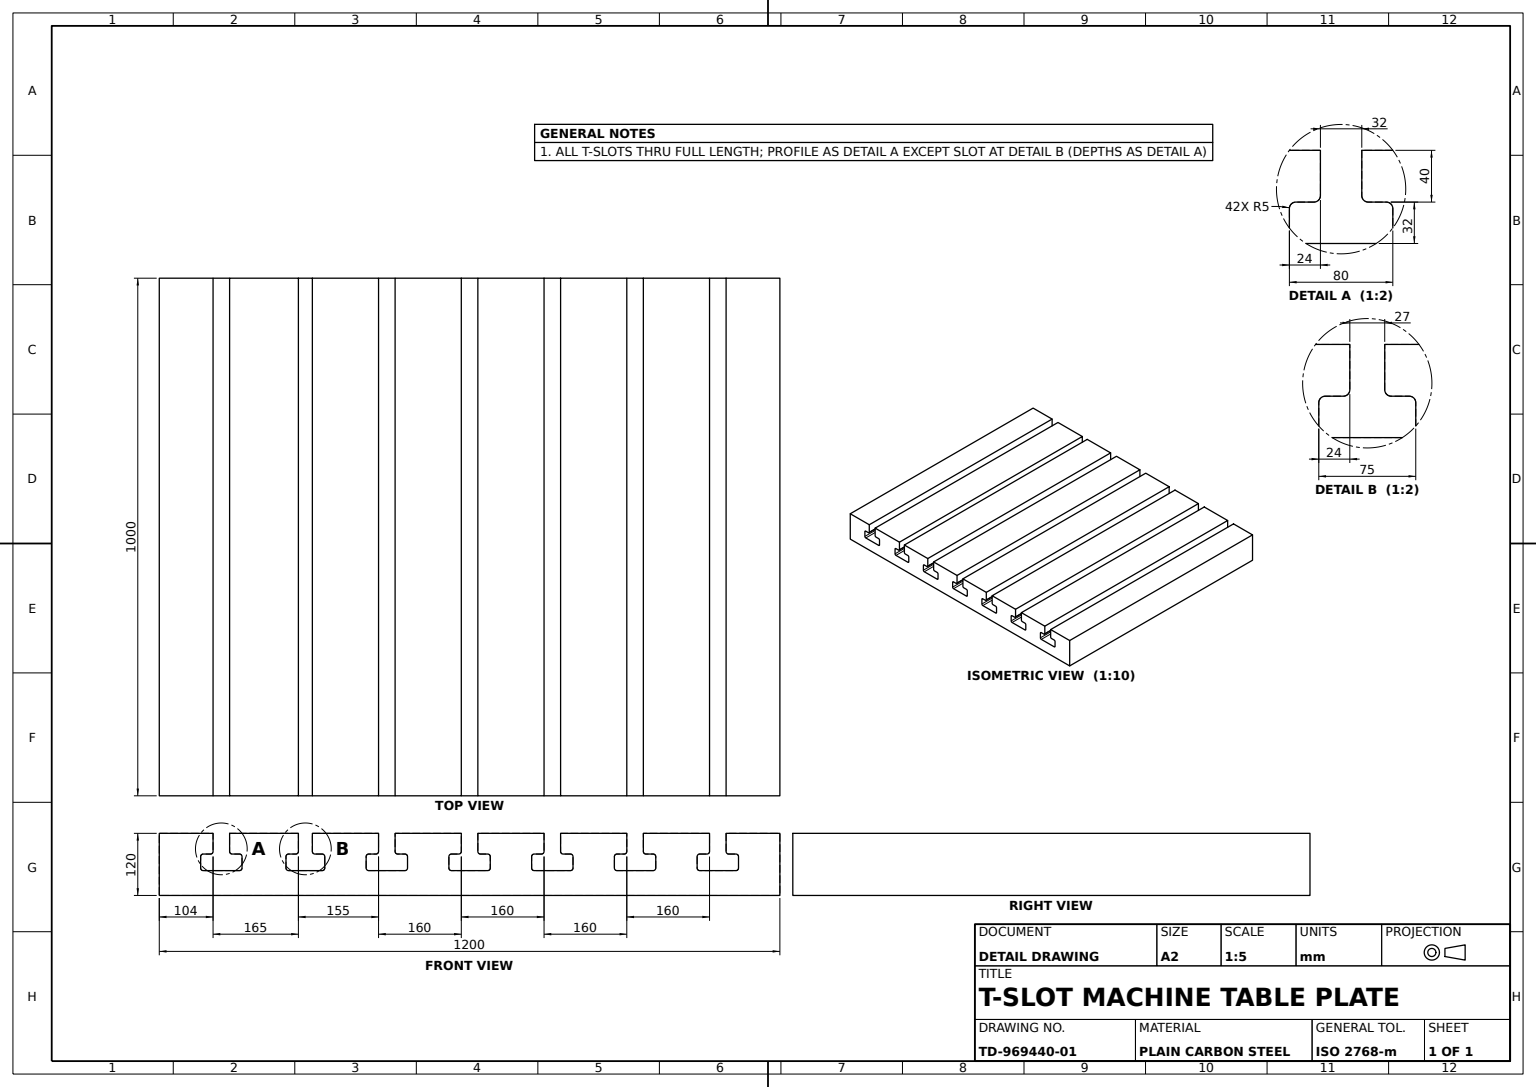
solid
v1 (104,1000,120)
v2 (104,1000,85)
e1 v1 v2 LINE
v3 (104,0,120)
e2 v1 v3 LINE
v4 (104,0,85)
e3 v3 v4 LINE
e4 v2 v4 LINE
face PLANE(AX(P(104,1000,0),D(-1,0,0),D(0,0,1))) rev [-e1 e2 e3 -e4]
v5 (1059,1000,80)
v6 (1059,0,80)
e5 v5 v6 LINE
v7 (1064,1000,85)
e6 v7 v5 CIRCLE(AX(P(1059,1000,85),D(0,1,0),D(0,0,-1)),5)
v8 (1064,0,85)
e7 v7 v8 LINE
e8 v8 v6 CIRCLE(AX(P(1059,0,85),D(0,1,0),D(0,0,-1)),5)
face CYL(AX(P(1059,1000,85),D(0,-1,0),D(0,0,-1)),5) [-e5 -e6 e7 e8]
v9 (885,1000,48)
v10 (885,0,48)
e9 v9 v10 LINE
v11 (955,0,48)
e10 v10 v11 LINE
v12 (955,1000,48)
e11 v12 v11 LINE
e12 v9 v12 LINE
face PLANE(AX(P(920,1000,48),D(0,0,-1),D(-1,0,0))) rev [e9 e10 -e11 -e12]
v13 (456,1000,85)
v14 (456,0,85)
e13 v13 v14 LINE
v15 (456,0,120)
e14 v14 v15 LINE
v16 (456,1000,120)
e15 v16 v15 LINE
e16 v13 v16 LINE
face PLANE(AX(P(456,1000,120),D(1,0,0),D(0,0,-1))) rev [e13 e14 -e15 -e16]
v17 (904,0,85)
v18 (899,0,80)
e17 v17 v18 CIRCLE(AX(P(899,0,85),D(0,1,0),D(0,0,-1)),5)
v19 (899,1000,80)
e18 v19 v18 LINE
v20 (904,1000,85)
e19 v20 v19 CIRCLE(AX(P(899,1000,85),D(0,1,0),D(0,0,-1)),5)
e20 v20 v17 LINE
face CYL(AX(P(899,1000,85),D(0,-1,0),D(0,0,-1)),5) [e17 -e18 -e19 e20]
v21 (85,0,80)
v22 (99,0,80)
e21 v21 v22 LINE
v23 (85,1000,80)
e22 v23 v21 LINE
v24 (99,1000,80)
e23 v23 v24 LINE
e24 v24 v22 LINE
face PLANE(AX(P(0,1000,80),D(0,0,-1),D(-1,0,0))) [-e21 -e22 e23 e24]
v25 (136,1000,85)
v26 (136,0,85)
e25 v25 v26 LINE
v27 (136,0,120)
e26 v27 v26 LINE
v28 (136,1000,120)
e27 v28 v27 LINE
e28 v28 v25 LINE
face PLANE(AX(P(136,1000,0),D(-1,0,0),D(0,0,1))) [e25 -e26 -e27 e28]
v29 (781,0,80)
v30 (776,0,85)
e29 v29 v30 CIRCLE(AX(P(781,0,85),D(0,1,0),D(0,0,1)),5)
v31 (776,1000,85)
e30 v31 v30 LINE
v32 (781,1000,80)
e31 v32 v31 CIRCLE(AX(P(781,1000,85),D(0,1,0),D(0,0,1)),5)
e32 v32 v29 LINE
face CYL(AX(P(781,1000,85),D(0,-1,0),D(0,0,-1)),5) [e29 -e30 -e31 e32]
v33 (904,1000,120)
e33 v33 v20 LINE
v34 (904,0,120)
e34 v33 v34 LINE
e35 v34 v17 LINE
face PLANE(AX(P(904,1000,85),D(-1,0,0),D(0,0,1))) rev [-e20 -e33 e34 e35]
v35 (936,1000,85)
v36 (936,1000,120)
e36 v35 v36 LINE
v37 (936,0,85)
e37 v35 v37 LINE
v38 (936,0,120)
e38 v37 v38 LINE
e39 v36 v38 LINE
face PLANE(AX(P(936,1000,120),D(1,0,0),D(0,0,-1))) rev [-e36 e37 e38 -e39]
v39 (1045,1000,48)
v40 (1045,0,48)
e40 v39 v40 LINE
v41 (1040,1000,53)
e41 v41 v39 CIRCLE(AX(P(1045,1000,53),D(0,-1,0),D(0,0,1)),5)
v42 (1040,0,53)
e42 v41 v42 LINE
e43 v42 v40 CIRCLE(AX(P(1045,0,53),D(0,-1,0),D(0,0,1)),5)
face CYL(AX(P(1045,1000,53),D(0,-1,0),D(0,0,-1)),5) rev [-e40 -e41 e42 e43]
v43 (424,1000,120)
v44 (424,0,120)
e44 v43 v44 LINE
v45 (424,0,85)
e45 v44 v45 LINE
v46 (424,1000,85)
e46 v46 v45 LINE
e47 v43 v46 LINE
face PLANE(AX(P(424,1000,120),D(-1,0,0),D(0,0,1))) rev [e44 e45 -e46 -e47]
v47 (776,0,120)
e48 v30 v47 LINE
v48 (776,1000,120)
e49 v48 v47 LINE
e50 v31 v48 LINE
face PLANE(AX(P(776,1000,120),D(1,0,0),D(0,0,-1))) rev [e30 e48 -e49 -e50]
e51 v24 v2 CIRCLE(AX(P(99,1000,85),D(0,-1,0),D(0,0,-1)),5)
e52 v22 v4 CIRCLE(AX(P(99,0,85),D(0,-1,0),D(0,0,-1)),5)
face CYL(AX(P(99,1000,85),D(0,-1,0),D(0,0,-1)),5) [-e24 e51 e4 -e52]
v49 (141,0,80)
v50 (155,0,80)
e53 v49 v50 LINE
v51 (141,1000,80)
e54 v51 v49 LINE
v52 (155,1000,80)
e55 v51 v52 LINE
e56 v52 v50 LINE
face PLANE(AX(P(0,1000,80),D(0,0,-1),D(-1,0,0))) [-e53 -e54 e55 e56]
v53 (0,0,0)
v54 (1200,0,0)
e57 v53 v54 LINE
v55 (0,1000,0)
e58 v55 v53 LINE
v56 (1200,1000,0)
e59 v56 v55 LINE
e60 v54 v56 LINE
face PLANE(AX(P(0,0,0),D(0,0,1),D(1,0,0))) rev [-e57 -e58 -e59 -e60]
v57 (160,1000,75)
v58 (160,0,75)
e61 v57 v58 LINE
v59 (160,1000,53)
e62 v59 v57 LINE
v60 (160,0,53)
e63 v59 v60 LINE
e64 v60 v58 LINE
face PLANE(AX(P(160,1000,0),D(1,0,0),D(0,0,-1))) rev [-e61 -e62 e63 e64]
v61 (960,1000,53)
e65 v12 v61 CIRCLE(AX(P(955,1000,53),D(0,-1,0),D(0,0,-1)),5)
v62 (960,0,53)
e66 v11 v62 CIRCLE(AX(P(955,0,53),D(0,-1,0),D(0,0,-1)),5)
e67 v61 v62 LINE
face CYL(AX(P(955,1000,53),D(0,-1,0),D(0,0,-1)),5) rev [-e65 e11 e66 -e67]
v63 (635,1000,48)
v64 (635,0,48)
e68 v63 v64 LINE
v65 (565,1000,48)
e69 v65 v63 LINE
v66 (565,0,48)
e70 v65 v66 LINE
e71 v66 v64 LINE
face PLANE(AX(P(600,1000,48),D(0,0,-1),D(-1,0,0))) rev [-e68 -e69 e70 e71]
v67 (955,0,80)
v68 (941,0,80)
e72 v67 v68 LINE
v69 (941,1000,80)
e73 v69 v68 LINE
v70 (955,1000,80)
e74 v70 v69 LINE
e75 v70 v67 LINE
face PLANE(AX(P(955,1000,80),D(0,0,1),D(1,0,0))) rev [e72 -e73 -e74 e75]
v71 (960,1000,75)
v72 (960,0,75)
e76 v71 v72 LINE
e77 v72 v67 CIRCLE(AX(P(955,0,75),D(0,-1,0),D(0,0,-1)),5)
e78 v71 v70 CIRCLE(AX(P(955,1000,75),D(0,-1,0),D(0,0,-1)),5)
face CYL(AX(P(955,1000,75),D(0,-1,0),D(0,0,-1)),5) rev [e76 e77 -e75 -e78]
v73 (640,0,53)
v74 (640,0,75)
e79 v73 v74 LINE
v75 (640,1000,75)
e80 v75 v74 LINE
v76 (640,1000,53)
e81 v76 v75 LINE
e82 v76 v73 LINE
face PLANE(AX(P(640,1000,53),D(1,0,0),D(0,0,-1))) rev [e79 -e80 -e81 e82]
e83 v57 v52 CIRCLE(AX(P(155,1000,75),D(0,-1,0),D(0,0,-1)),5)
e84 v58 v50 CIRCLE(AX(P(155,0,75),D(0,-1,0),D(0,0,-1)),5)
face CYL(AX(P(155,1000,75),D(0,-1,0),D(0,0,-1)),5) rev [-e56 -e83 e61 e84]
v77 (480,1000,53)
v78 (480,0,53)
e85 v77 v78 LINE
v79 (480,0,75)
e86 v78 v79 LINE
v80 (480,1000,75)
e87 v80 v79 LINE
e88 v77 v80 LINE
face PLANE(AX(P(480,1000,53),D(1,0,0),D(0,0,-1))) rev [e85 e86 -e87 -e88]
e89 v49 v26 CIRCLE(AX(P(141,0,85),D(0,1,0),D(0,0,-1)),5)
e90 v51 v25 CIRCLE(AX(P(141,1000,85),D(0,1,0),D(0,0,-1)),5)
face CYL(AX(P(141,1000,85),D(0,-1,0),D(0,0,-1)),5) [e54 e89 -e25 -e90]
v81 (795,1000,80)
v82 (795,0,80)
e91 v81 v82 LINE
e92 v82 v29 LINE
e93 v81 v32 LINE
face PLANE(AX(P(795,1000,80),D(0,0,1),D(1,0,0))) rev [e91 e92 -e32 -e93]
v83 (245,1000,75)
v84 (245,1000,53)
e94 v83 v84 LINE
v85 (245,0,75)
e95 v83 v85 LINE
v86 (245,0,53)
e96 v85 v86 LINE
e97 v84 v86 LINE
face PLANE(AX(P(245,1000,53),D(-1,0,0),D(0,0,1))) rev [-e94 e95 e96 -e97]
v87 (1045,0,80)
v88 (1040,0,75)
e98 v87 v88 CIRCLE(AX(P(1045,0,75),D(0,-1,0),D(0,0,-1)),5)
v89 (1040,1000,75)
e99 v89 v88 LINE
v90 (1045,1000,80)
e100 v90 v89 CIRCLE(AX(P(1045,1000,75),D(0,-1,0),D(0,0,-1)),5)
e101 v90 v87 LINE
face CYL(AX(P(1045,1000,75),D(0,-1,0),D(0,0,-1)),5) rev [e98 -e99 -e100 e101]
v91 (880,1000,75)
v92 (880,1000,53)
e102 v91 v92 LINE
v93 (880,0,75)
e103 v91 v93 LINE
v94 (880,0,53)
e104 v93 v94 LINE
e105 v92 v94 LINE
face PLANE(AX(P(880,1000,53),D(-1,0,0),D(0,0,1))) rev [-e102 e103 e104 -e105]
v95 (296,1000,120)
e106 v43 v95 LINE
v96 (296,0,120)
e107 v95 v96 LINE
e108 v96 v44 LINE
face PLANE(AX(P(0,0,120),D(0,0,1),D(1,0,0))) [-e44 e106 e107 e108]
v97 (885,0,80)
e109 v97 v93 CIRCLE(AX(P(885,0,75),D(0,-1,0),D(0,0,-1)),5)
v98 (885,1000,80)
e110 v98 v91 CIRCLE(AX(P(885,1000,75),D(0,-1,0),D(0,0,-1)),5)
e111 v98 v97 LINE
face CYL(AX(P(885,1000,75),D(0,-1,0),D(0,0,-1)),5) rev [e109 -e103 -e110 e111]
v99 (1115,1000,48)
v100 (1120,1000,53)
e112 v99 v100 CIRCLE(AX(P(1115,1000,53),D(0,-1,0),D(0,0,-1)),5)
v101 (1115,0,48)
e113 v99 v101 LINE
v102 (1120,0,53)
e114 v101 v102 CIRCLE(AX(P(1115,0,53),D(0,-1,0),D(0,0,-1)),5)
e115 v100 v102 LINE
face CYL(AX(P(1115,1000,53),D(0,-1,0),D(0,0,-1)),5) rev [-e112 e113 e114 -e115]
v103 (461,0,80)
e116 v103 v14 CIRCLE(AX(P(461,0,85),D(0,1,0),D(0,0,1)),5)
v104 (461,1000,80)
e117 v104 v13 CIRCLE(AX(P(461,1000,85),D(0,1,0),D(0,0,1)),5)
e118 v104 v103 LINE
face CYL(AX(P(461,1000,85),D(0,-1,0),D(0,0,-1)),5) [e116 -e13 -e117 e118]
v105 (0,0,120)
e119 v105 v53 LINE
v106 (0,1000,120)
e120 v106 v105 LINE
e121 v106 v55 LINE
face PLANE(AX(P(0,1000,120),D(1,0,0),D(0,0,-1))) rev [e58 -e119 -e120 e121]
v107 (80,1000,75)
v108 (80,0,75)
e122 v107 v108 LINE
e123 v23 v107 CIRCLE(AX(P(85,1000,75),D(0,-1,0),D(0,0,-1)),5)
e124 v21 v108 CIRCLE(AX(P(85,0,75),D(0,-1,0),D(0,0,-1)),5)
face CYL(AX(P(85,1000,75),D(0,-1,0),D(0,0,-1)),5) rev [-e122 -e123 e22 e124]
e125 v64 v73 CIRCLE(AX(P(635,0,53),D(0,-1,0),D(0,0,-1)),5)
e126 v63 v76 CIRCLE(AX(P(635,1000,53),D(0,-1,0),D(0,0,-1)),5)
face CYL(AX(P(635,1000,53),D(0,-1,0),D(0,0,-1)),5) rev [e68 e125 -e82 -e126]
v109 (584,0,120)
e127 v15 v109 LINE
v110 (584,1000,120)
e128 v110 v109 LINE
e129 v110 v16 LINE
face PLANE(AX(P(0,0,120),D(0,0,1),D(1,0,0))) [e15 e127 -e128 e129]
e130 v94 v10 CIRCLE(AX(P(885,0,53),D(0,-1,0),D(0,0,1)),5)
e131 v92 v9 CIRCLE(AX(P(885,1000,53),D(0,-1,0),D(0,0,1)),5)
face CYL(AX(P(885,1000,53),D(0,-1,0),D(0,0,-1)),5) rev [e105 e130 -e9 -e131]
v111 (800,1000,53)
v112 (800,1000,75)
e132 v111 v112 LINE
v113 (800,0,53)
e133 v111 v113 LINE
v114 (800,0,75)
e134 v113 v114 LINE
e135 v112 v114 LINE
face PLANE(AX(P(800,1000,53),D(1,0,0),D(0,0,-1))) rev [-e132 e133 e134 -e135]
v115 (1120,0,75)
v116 (1115,0,80)
e136 v115 v116 CIRCLE(AX(P(1115,0,75),D(0,-1,0),D(0,0,-1)),5)
v117 (1115,1000,80)
e137 v117 v116 LINE
v118 (1120,1000,75)
e138 v118 v117 CIRCLE(AX(P(1115,1000,75),D(0,-1,0),D(0,0,-1)),5)
e139 v118 v115 LINE
face CYL(AX(P(1115,1000,75),D(0,-1,0),D(0,0,-1)),5) rev [e136 -e137 -e138 e139]
v119 (725,1000,48)
v120 (725,0,48)
e140 v119 v120 LINE
v121 (795,0,48)
e141 v120 v121 LINE
v122 (795,1000,48)
e142 v122 v121 LINE
e143 v119 v122 LINE
face PLANE(AX(P(760,1000,48),D(0,0,-1),D(-1,0,0))) rev [e140 e141 -e142 -e143]
v123 (739,1000,80)
v124 (739,0,80)
e144 v123 v124 LINE
v125 (725,0,80)
e145 v124 v125 LINE
v126 (725,1000,80)
e146 v126 v125 LINE
e147 v123 v126 LINE
face PLANE(AX(P(725,1000,80),D(0,0,1),D(1,0,0))) rev [e144 e145 -e146 -e147]
v127 (1200,0,120)
v128 (1200,1000,120)
e148 v127 v128 LINE
e149 v127 v54 LINE
e150 v128 v56 LINE
face PLANE(AX(P(1200,0,120),D(-1,0,0),D(0,0,1))) rev [-e148 e149 e60 -e150]
v129 (405,1000,80)
v130 (405,0,80)
e151 v129 v130 LINE
v131 (400,0,75)
e152 v130 v131 CIRCLE(AX(P(405,0,75),D(0,-1,0),D(0,0,-1)),5)
v132 (400,1000,75)
e153 v132 v131 LINE
e154 v129 v132 CIRCLE(AX(P(405,1000,75),D(0,-1,0),D(0,0,-1)),5)
face CYL(AX(P(405,1000,75),D(0,-1,0),D(0,0,-1)),5) rev [e151 e152 -e153 -e154]
v133 (744,1000,120)
v134 (744,1000,85)
e155 v133 v134 LINE
v135 (744,0,120)
e156 v133 v135 LINE
v136 (744,0,85)
e157 v135 v136 LINE
e158 v134 v136 LINE
face PLANE(AX(P(744,1000,120),D(-1,0,0),D(0,0,1))) rev [-e155 e156 e157 -e158]
v137 (400,0,53)
e159 v131 v137 LINE
v138 (400,1000,53)
e160 v138 v137 LINE
e161 v132 v138 LINE
face PLANE(AX(P(400,1000,53),D(-1,0,0),D(0,0,1))) rev [e153 e159 -e160 -e161]
v139 (419,0,80)
e162 v45 v139 CIRCLE(AX(P(419,0,85),D(0,1,0),D(0,0,-1)),5)
v140 (419,1000,80)
e163 v140 v139 LINE
e164 v46 v140 CIRCLE(AX(P(419,1000,85),D(0,1,0),D(0,0,-1)),5)
face CYL(AX(P(419,1000,85),D(0,-1,0),D(0,0,-1)),5) [e162 -e163 -e164 e46]
v141 (475,1000,48)
e165 v141 v77 CIRCLE(AX(P(475,1000,53),D(0,-1,0),D(0,0,-1)),5)
v142 (475,0,48)
e166 v141 v142 LINE
e167 v142 v78 CIRCLE(AX(P(475,0,53),D(0,-1,0),D(0,0,-1)),5)
face CYL(AX(P(475,1000,53),D(0,-1,0),D(0,0,-1)),5) rev [-e165 e166 e167 -e85]
v143 (475,0,80)
e168 v143 v103 LINE
v144 (475,1000,80)
e169 v144 v104 LINE
e170 v144 v143 LINE
face PLANE(AX(P(475,1000,80),D(0,0,1),D(1,0,0))) rev [e168 -e118 -e169 e170]
v145 (720,1000,75)
v146 (720,0,75)
e171 v145 v146 LINE
v147 (720,0,53)
e172 v146 v147 LINE
v148 (720,1000,53)
e173 v148 v147 LINE
e174 v145 v148 LINE
face PLANE(AX(P(720,1000,53),D(-1,0,0),D(0,0,1))) rev [e171 e172 -e173 -e174]
e175 v140 v129 LINE
e176 v139 v130 LINE
face PLANE(AX(P(405,1000,80),D(0,0,1),D(1,0,0))) rev [-e151 -e175 e163 e176]
v149 (301,1000,80)
v150 (301,0,80)
e177 v149 v150 LINE
v151 (296,0,85)
e178 v150 v151 CIRCLE(AX(P(301,0,85),D(0,1,0),D(0,0,1)),5)
v152 (296,1000,85)
e179 v152 v151 LINE
e180 v149 v152 CIRCLE(AX(P(301,1000,85),D(0,1,0),D(0,0,1)),5)
face CYL(AX(P(301,1000,85),D(0,-1,0),D(0,0,-1)),5) [e177 e178 -e179 -e180]
e181 v40 v101 LINE
e182 v39 v99 LINE
face PLANE(AX(P(1080,1000,48),D(0,0,-1),D(-1,0,0))) rev [e40 e181 -e113 -e182]
e183 v112 v81 CIRCLE(AX(P(795,1000,75),D(0,-1,0),D(0,0,-1)),5)
e184 v114 v82 CIRCLE(AX(P(795,0,75),D(0,-1,0),D(0,0,-1)),5)
face CYL(AX(P(795,1000,75),D(0,-1,0),D(0,0,-1)),5) rev [-e183 e135 e184 -e91]
e185 v18 v97 LINE
e186 v19 v98 LINE
face PLANE(AX(P(885,1000,80),D(0,0,1),D(1,0,0))) rev [e18 e185 -e111 -e186]
e187 v125 v146 CIRCLE(AX(P(725,0,75),D(0,-1,0),D(0,0,1)),5)
e188 v126 v145 CIRCLE(AX(P(725,1000,75),D(0,-1,0),D(0,0,1)),5)
face CYL(AX(P(725,1000,75),D(0,-1,0),D(0,0,-1)),5) rev [e187 -e171 -e188 e146]
v153 (405,1000,48)
v154 (405,0,48)
e189 v153 v154 LINE
e190 v138 v153 CIRCLE(AX(P(405,1000,53),D(0,-1,0),D(0,0,1)),5)
e191 v137 v154 CIRCLE(AX(P(405,0,53),D(0,-1,0),D(0,0,1)),5)
face CYL(AX(P(405,1000,53),D(0,-1,0),D(0,0,-1)),5) rev [-e189 -e190 e160 e191]
e192 v47 v34 LINE
e193 v33 v48 LINE
face PLANE(AX(P(0,0,120),D(0,0,1),D(1,0,0))) [e49 e192 -e34 e193]
e194 v152 v95 LINE
e195 v151 v96 LINE
face PLANE(AX(P(296,1000,120),D(1,0,0),D(0,0,-1))) rev [-e194 e179 e195 -e107]
v155 (1096,1000,120)
v156 (1096,0,120)
e196 v155 v156 LINE
v157 (1096,1000,85)
e197 v157 v155 LINE
v158 (1096,0,85)
e198 v157 v158 LINE
e199 v158 v156 LINE
face PLANE(AX(P(1096,1000,120),D(1,0,0),D(0,0,-1))) rev [-e196 -e197 e198 e199]
v159 (80,0,53)
e200 v108 v159 LINE
v160 (80,1000,53)
e201 v160 v159 LINE
e202 v107 v160 LINE
face PLANE(AX(P(80,1000,0),D(-1,0,0),D(0,0,1))) rev [e200 -e201 -e202 e122]
e203 v147 v120 CIRCLE(AX(P(725,0,53),D(0,-1,0),D(0,0,1)),5)
e204 v148 v119 CIRCLE(AX(P(725,1000,53),D(0,-1,0),D(0,0,1)),5)
face CYL(AX(P(725,1000,53),D(0,-1,0),D(0,0,-1)),5) rev [e173 e203 -e140 -e204]
v161 (315,1000,80)
v162 (315,0,80)
e205 v161 v162 LINE
e206 v162 v150 LINE
e207 v161 v149 LINE
face PLANE(AX(P(315,1000,80),D(0,0,1),D(1,0,0))) rev [e205 e206 -e177 -e207]
v163 (315,0,48)
v164 (320,0,53)
e208 v163 v164 CIRCLE(AX(P(315,0,53),D(0,-1,0),D(0,0,-1)),5)
v165 (320,1000,53)
e209 v165 v164 LINE
v166 (315,1000,48)
e210 v166 v165 CIRCLE(AX(P(315,1000,53),D(0,-1,0),D(0,0,-1)),5)
e211 v166 v163 LINE
face CYL(AX(P(315,1000,53),D(0,-1,0),D(0,0,-1)),5) rev [e208 -e209 -e210 e211]
v167 (269,0,120)
v168 (269,0,85)
e212 v167 v168 LINE
v169 (269,1000,85)
e213 v169 v168 LINE
v170 (269,1000,120)
e214 v170 v169 LINE
e215 v170 v167 LINE
face PLANE(AX(P(269,1000,85),D(-1,0,0),D(0,0,1))) rev [e212 -e213 -e214 e215]
v171 (565,1000,80)
v172 (565,0,80)
e216 v171 v172 LINE
v173 (579,1000,80)
e217 v173 v171 LINE
v174 (579,0,80)
e218 v173 v174 LINE
e219 v174 v172 LINE
face PLANE(AX(P(565,1000,80),D(0,0,1),D(1,0,0))) rev [-e216 -e217 e218 e219]
v175 (250,1000,80)
v176 (250,0,80)
e220 v175 v176 LINE
v177 (264,1000,80)
e221 v177 v175 LINE
v178 (264,0,80)
e222 v177 v178 LINE
e223 v178 v176 LINE
face PLANE(AX(P(250,1000,80),D(0,0,1),D(1,0,0))) rev [-e220 -e221 e222 e223]
e224 v134 v123 CIRCLE(AX(P(739,1000,85),D(0,1,0),D(0,0,-1)),5)
e225 v136 v124 CIRCLE(AX(P(739,0,85),D(0,1,0),D(0,0,-1)),5)
face CYL(AX(P(739,1000,85),D(0,-1,0),D(0,0,-1)),5) [-e144 -e224 e158 e225]
v179 (250,0,48)
e226 v86 v179 CIRCLE(AX(P(250,0,53),D(0,-1,0),D(0,0,1)),5)
v180 (250,1000,48)
e227 v180 v179 LINE
e228 v84 v180 CIRCLE(AX(P(250,1000,53),D(0,-1,0),D(0,0,1)),5)
face CYL(AX(P(250,1000,53),D(0,-1,0),D(0,0,-1)),5) rev [e97 e226 -e227 -e228]
v181 (616,1000,85)
v182 (616,0,85)
e229 v181 v182 LINE
v183 (621,1000,80)
e230 v183 v181 CIRCLE(AX(P(621,1000,85),D(0,1,0),D(0,0,1)),5)
v184 (621,0,80)
e231 v183 v184 LINE
e232 v184 v182 CIRCLE(AX(P(621,0,85),D(0,1,0),D(0,0,1)),5)
face CYL(AX(P(621,1000,85),D(0,-1,0),D(0,0,-1)),5) [-e229 -e230 e231 e232]
v185 (155,0,48)
e233 v185 v60 CIRCLE(AX(P(155,0,53),D(0,-1,0),D(0,0,-1)),5)
v186 (155,1000,48)
e234 v186 v59 CIRCLE(AX(P(155,1000,53),D(0,-1,0),D(0,0,-1)),5)
e235 v186 v185 LINE
face CYL(AX(P(155,1000,53),D(0,-1,0),D(0,0,-1)),5) rev [e233 -e63 -e234 e235]
e236 v122 v111 CIRCLE(AX(P(795,1000,53),D(0,-1,0),D(0,0,-1)),5)
e237 v121 v113 CIRCLE(AX(P(795,0,53),D(0,-1,0),D(0,0,-1)),5)
face CYL(AX(P(795,1000,53),D(0,-1,0),D(0,0,-1)),5) rev [-e133 -e236 e142 e237]
v187 (320,0,75)
e238 v187 v162 CIRCLE(AX(P(315,0,75),D(0,-1,0),D(0,0,-1)),5)
e239 v164 v187 LINE
e240 v179 v163 LINE
e241 v176 v85 CIRCLE(AX(P(250,0,75),D(0,-1,0),D(0,0,-1)),5)
e242 v168 v178 CIRCLE(AX(P(264,0,85),D(0,1,0),D(0,0,-1)),5)
e243 v27 v167 LINE
v188 (85,0,48)
e244 v188 v185 LINE
e245 v188 v159 CIRCLE(AX(P(85,0,53),D(0,1,0),D(0,0,-1)),5)
e246 v105 v3 LINE
e247 v156 v127 LINE
v189 (1101,0,80)
e248 v189 v158 CIRCLE(AX(P(1101,0,85),D(0,1,0),D(0,0,1)),5)
e249 v116 v189 LINE
e250 v102 v115 LINE
e251 v88 v42 LINE
e252 v6 v87 LINE
v190 (1064,0,120)
e253 v190 v8 LINE
e254 v38 v190 LINE
e255 v68 v37 CIRCLE(AX(P(941,0,85),D(0,1,0),D(0,0,1)),5)
e256 v62 v72 LINE
v191 (616,0,120)
e257 v191 v135 LINE
e258 v182 v191 LINE
v192 (635,0,80)
e259 v192 v184 LINE
e260 v74 v192 CIRCLE(AX(P(635,0,75),D(0,-1,0),D(0,0,-1)),5)
v193 (560,0,53)
e261 v193 v66 CIRCLE(AX(P(565,0,53),D(0,-1,0),D(0,0,1)),5)
v194 (560,0,75)
e262 v194 v193 LINE
e263 v172 v194 CIRCLE(AX(P(565,0,75),D(0,-1,0),D(0,0,1)),5)
v195 (584,0,85)
e264 v195 v174 CIRCLE(AX(P(579,0,85),D(0,1,0),D(0,0,-1)),5)
e265 v109 v195 LINE
e266 v79 v143 CIRCLE(AX(P(475,0,75),D(0,-1,0),D(0,0,-1)),5)
e267 v154 v142 LINE
face PLANE(AX(P(0,0,120),D(0,1,0),D(0,0,1))) rev [-e195 -e178 -e206 -e238 -e239 -e208 -e240 -e226 -e96 -e241 -e223 -e242 -e212 -e243 e26 -e89 e53 -e84 -e64 -e233 -e244 e245 -e200 -e124 e21 e52 -e3 -e246 e119 e57 -e149 -e247 -e199 -e248 -e249 -e136 -e250 -e114 -e181 -e43 -e251 -e98 -e252 -e8 -e253 -e254 -e38 -e255 -e72 -e77 -e256 -e66 -e10 -e130 -e104 -e109 -e185 -e17 -e35 -e192 -e48 -e29 -e92 -e184 -e134 -e237 -e141 -e203 -e172 -e187 -e145 -e225 -e157 -e257 -e258 -e232 -e259 -e260 -e79 -e125 -e71 -e261 -e262 -e263 -e219 -e264 -e265 -e127 -e14 -e116 -e168 -e266 -e86 -e167 -e267 -e191 -e159 -e152 -e176 -e162 -e45 -e108]
e268 v69 v35 CIRCLE(AX(P(941,1000,85),D(0,1,0),D(0,0,1)),5)
face CYL(AX(P(941,1000,85),D(0,-1,0),D(0,0,-1)),5) [e255 -e37 -e268 e73]
v196 (616,1000,120)
e269 v196 v191 LINE
e270 v181 v196 LINE
face PLANE(AX(P(616,1000,120),D(1,0,0),D(0,0,-1))) rev [-e269 -e270 e229 e258]
e271 v61 v71 LINE
face PLANE(AX(P(960,1000,53),D(1,0,0),D(0,0,-1))) rev [-e271 e67 e256 -e76]
e272 v80 v144 CIRCLE(AX(P(475,1000,75),D(0,-1,0),D(0,0,-1)),5)
v197 (584,1000,85)
e273 v110 v197 LINE
e274 v197 v173 CIRCLE(AX(P(579,1000,85),D(0,1,0),D(0,0,-1)),5)
v198 (560,1000,75)
e275 v171 v198 CIRCLE(AX(P(565,1000,75),D(0,-1,0),D(0,0,1)),5)
v199 (560,1000,53)
e276 v198 v199 LINE
e277 v199 v65 CIRCLE(AX(P(565,1000,53),D(0,-1,0),D(0,0,1)),5)
v200 (635,1000,80)
e278 v75 v200 CIRCLE(AX(P(635,1000,75),D(0,-1,0),D(0,0,-1)),5)
e279 v200 v183 LINE
e280 v133 v196 LINE
v201 (1064,1000,120)
e281 v201 v36 LINE
e282 v201 v7 LINE
e283 v5 v90 LINE
e284 v89 v41 LINE
e285 v100 v118 LINE
v202 (1101,1000,80)
e286 v117 v202 LINE
e287 v202 v157 CIRCLE(AX(P(1101,1000,85),D(0,1,0),D(0,0,1)),5)
e288 v128 v155 LINE
e289 v1 v106 LINE
v203 (85,1000,48)
e290 v203 v160 CIRCLE(AX(P(85,1000,53),D(0,1,0),D(0,0,-1)),5)
e291 v203 v186 LINE
e292 v170 v28 LINE
e293 v169 v177 CIRCLE(AX(P(264,1000,85),D(0,1,0),D(0,0,-1)),5)
e294 v175 v83 CIRCLE(AX(P(250,1000,75),D(0,-1,0),D(0,0,-1)),5)
e295 v180 v166 LINE
v204 (320,1000,75)
e296 v165 v204 LINE
e297 v204 v161 CIRCLE(AX(P(315,1000,75),D(0,-1,0),D(0,0,-1)),5)
e298 v153 v141 LINE
face PLANE(AX(P(1200,1000,120),D(0,-1,0),D(0,0,-1))) rev [e165 e88 e272 e169 e117 e16 -e129 e273 e274 e217 e275 e276 e277 e69 e126 e81 e278 e279 e230 e270 -e280 e155 e224 e147 e188 e174 e204 e143 e236 e132 e183 e93 e31 e50 -e193 e33 e19 e186 e110 e102 e131 e12 e65 e271 e78 e74 e268 e36 -e281 e282 e6 e283 e100 e284 e41 e182 e112 e285 e138 e286 e287 e197 -e288 e150 e59 -e121 -e289 e1 -e51 -e23 e123 e202 -e290 e291 e234 e62 e83 -e55 e90 -e28 -e292 e214 e293 e221 e294 e94 e228 e295 e210 e296 e297 e207 e180 e194 -e106 e47 e164 e175 e154 e161 e190 e298]
e299 v198 v194 LINE
e300 v199 v193 LINE
face PLANE(AX(P(560,1000,53),D(-1,0,0),D(0,0,1))) rev [e299 e262 -e300 -e276]
face PLANE(AX(P(0,0,120),D(0,0,1),D(1,0,0))) [e280 e269 e257 -e156]
face PLANE(AX(P(0,0,120),D(0,0,1),D(1,0,0))) [e246 -e2 e289 e120]
face CYL(AX(P(475,1000,75),D(0,-1,0),D(0,0,-1)),5) rev [-e170 -e272 e87 e266]
face CYL(AX(P(565,1000,75),D(0,-1,0),D(0,0,-1)),5) rev [-e275 e216 e263 -e299]
face CYL(AX(P(250,1000,75),D(0,-1,0),D(0,0,-1)),5) rev [-e95 -e294 e220 e241]
face PLANE(AX(P(0,0,120),D(0,0,1),D(1,0,0))) [e288 e196 e247 e148]
e301 v201 v190 LINE
face PLANE(AX(P(0,0,120),D(0,0,1),D(1,0,0))) [e281 e39 e254 -e301]
e302 v197 v195 LINE
face CYL(AX(P(579,1000,85),D(0,-1,0),D(0,0,-1)),5) [-e218 -e274 e302 e264]
e303 v203 v188 LINE
face PLANE(AX(P(0,1000,48),D(0,0,-1),D(-1,0,0))) rev [e244 -e235 -e291 e303]
face CYL(AX(P(565,1000,53),D(0,-1,0),D(0,0,-1)),5) rev [-e70 -e277 e300 e261]
face PLANE(AX(P(584,1000,120),D(-1,0,0),D(0,0,1))) rev [-e302 -e273 e128 e265]
e304 v200 v192 LINE
face PLANE(AX(P(635,1000,80),D(0,0,1),D(1,0,0))) rev [e304 e259 -e231 -e279]
e305 v204 v187 LINE
face PLANE(AX(P(320,1000,53),D(1,0,0),D(0,0,-1))) rev [e209 e239 -e305 -e296]
face PLANE(AX(P(1120,1000,53),D(1,0,0),D(0,0,-1))) rev [e250 -e139 -e285 e115]
face PLANE(AX(P(1045,1000,80),D(0,0,1),D(1,0,0))) rev [e252 -e101 -e283 e5]
face PLANE(AX(P(1064,1000,85),D(-1,0,0),D(0,0,1))) rev [-e7 -e282 e301 e253]
face PLANE(AX(P(280,1000,48),D(0,0,-1),D(-1,0,0))) rev [-e295 e227 e240 -e211]
face CYL(AX(P(635,1000,75),D(0,-1,0),D(0,0,-1)),5) rev [e260 -e304 -e278 e80]
e306 v202 v189 LINE
face CYL(AX(P(1101,1000,85),D(0,-1,0),D(0,0,-1)),5) [-e287 e306 e248 -e198]
face CYL(AX(P(85,1000,53),D(0,-1,0),D(0,0,-1)),5) rev [e290 e201 -e245 -e303]
face PLANE(AX(P(0,0,120),D(0,0,1),D(1,0,0))) [e292 e27 e243 -e215]
face PLANE(AX(P(1115,1000,80),D(0,0,1),D(1,0,0))) rev [-e306 -e286 e137 e249]
face CYL(AX(P(264,1000,85),D(0,-1,0),D(0,0,-1)),5) [-e293 e213 e242 -e222]
face PLANE(AX(P(440,1000,48),D(0,0,-1),D(-1,0,0))) rev [e189 e267 -e166 -e298]
face PLANE(AX(P(1040,1000,53),D(-1,0,0),D(0,0,1))) rev [e99 e251 -e42 -e284]
face CYL(AX(P(315,1000,75),D(0,-1,0),D(0,0,-1)),5) rev [-e205 -e297 e305 e238]
